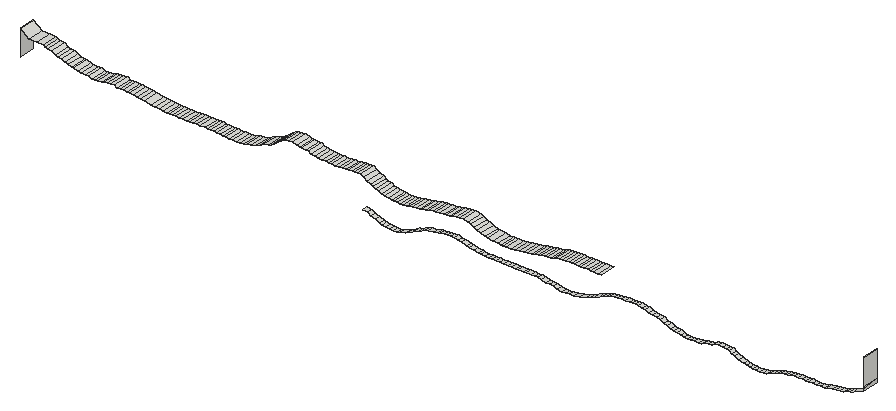
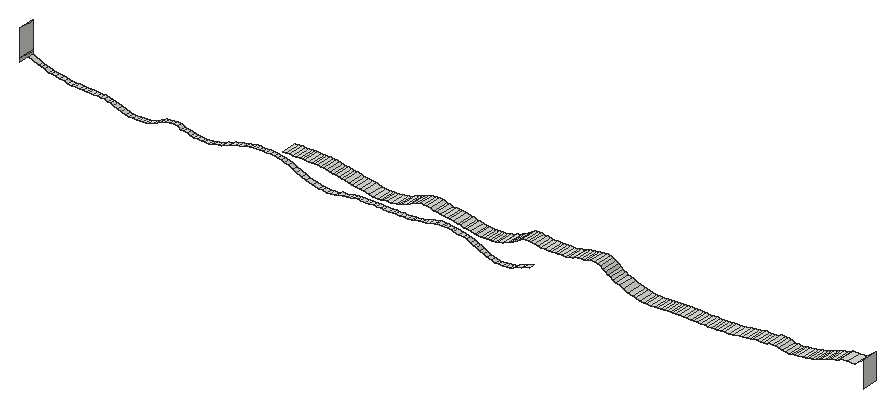
# SketchUp Ruby script. Lengths in inches.
U = 1.inch
M = Sketchup.active_model
def pt(a) = Geom::Point3d.new(a.map { |v| v * U })
def face(e, loops, mat)
  f = e.add_face(loops[0].map { |a| pt(a) })
  loops[1..].each { |l| e.add_face(l.map { |a| pt(a) }).erase! }
  f.material = f.back_material = mat if mat
  f
end
# faces: each face lists its corners as indices into pts; further lists are holes
def faces(e, pts, list, mat = nil) = list.each { |f| face(e, (f[0].is_a?(Array) ? f : [f]).map { |l| l.map { |i| pts[i] } }, mat) }
# xy, xz, yz: faces in a plane at the given z, y or x. An outline is a flat list of corners, or four numbers for a rectangle; further outlines are holes
def ring(l) = l.size == 4 ? [[l[0], l[1]], [l[2], l[1]], [l[2], l[3]], [l[0], l[3]]] : l.each_slice(2).to_a
def flat(e, list, mat, &to3) = list.each { |f| face(e, (f[0].is_a?(Array) ? f : [f]).map { |l| ring(l).map { |u, v| to3.(u, v) } }, mat) }
def xy(e, z, list, mat = nil) = flat(e, list, mat) { |x, y| [x, y, z] }
def xz(e, y, list, mat = nil) = flat(e, list, mat) { |x, z| [x, y, z] }
def yz(e, x, list, mat = nil) = flat(e, list, mat) { |y, z| [x, y, z] }
def lines(e, pts, list) = list.each { |a, b| e.add_line(pt(pts[a]), pt(pts[b])) }
# prism: a flat outline (further loops are holes) pulled along v
def prism(e, loops, v, mat = nil)
  f = face(e, loops, mat); d = Geom::Vector3d.new(v.map { |x| x * U })
  f.pushpull(f.normal.samedirection?(d) ? d.length : -d.length)
end
def box(e, o, s, mat = nil) = prism(e, [[o, [o[0] + s[0], o[1], o[2]], [o[0] + s[0], o[1] + s[1], o[2]], [o[0], o[1] + s[1], o[2]]]], [0, 0, s[2]], mat)
def at(x, y, z, deg = 0) = Geom::Transformation.translation(pt([x, y, z])) * Geom::Transformation.rotation(ORIGIN, Z_AXIS, deg.degrees)
def axes(o, x, y, z) = Geom::Transformation.new([*x, 0, *y, 0, *z, 0, *pt(o).to_a, 1])
def part(name) = M.definitions.add(name)
# library, detail: a bought-in or finely detailed component or shape, given as its bounding box
def library(name, o, s) = part(name).tap { |d| box(d.entities, o, s) }
def detail(e, o, s) = box(e.add_group.entities, o, s)
def put(e, d, t, mat = nil) = e.add_instance(d, t).tap { |i| i.material = mat if mat }
def group(e, t, mat = nil) = e.add_group.tap { |g| g.transformation = t; g.material = mat if mat }.entities
root = M.entities
xy(root,238.18,[[3012.28,2401.37,3012.96,2402.3]])
xy(root,238.62,[[2978.81,2401.37,2979.58,2402.3],[2979.58,2401.37,2980.21,2402.3],[2980.21,2401.37,2980.97,2402.3],[2980.97,2401.37,2981.59,2402.3],[2981.59,2401.37,2982.44,2402.3],
  [2982.44,2401.37,2983.08,2402.3],[2983.08,2401.37,2983.7,2402.3]])
xy(root,238.625,[[2977.39,2401.37,2978.25,2402.3]])
xy(root,238.89,[[3033.2,2401.37,3033.88,2402.3]])
xy(root,238.9,[[3034.64,2401.37,3035.26,2402.3],[3035.26,2401.37,3036.03,2402.3]])
xy(root,240.43,[[3001.48,2401.37,3002.05,2402.3]])
xy(root,241.68,[[2919.53,2401.37,2920.12,2404.3]])
xy(root,241.75,[[2921.88,2401.37,2922.75,2404.3],[2922.75,2401.37,2923.37,2404.3],[2923.37,2401.37,2923.88,2404.3]])
xy(root,243.05,[[2994.54,2401.37,2995.22,2404.3]])
xy(root,243.07,[[2992.6875,2401.37,2993.27,2404.3]])
xy(root,243.09,[[2989.375,2401.37,2989.9,2404.3],[2989.9,2401.37,2990.42,2404.3],[2990.42,2401.37,2991.08,2404.3],[2991.08,2401.37,2991.53,2404.3]])
yz(root,2889.09,[[2401.37,241.52,2404.3,246.2]])
yz(root,3043.1,[[2401.37,240.89,2401.37,241.29,2404.3,241.52,2404.3,240.89],[2401.37,241.29,2404.3,241.52,2401.37,241.52],[2401.37,241.52,2401.37,246.27,2402.0625,246.36,2404.3,246.43,2404.3,241.52],[2401.37,246.27,2401.37,246.43,2404.3,246.43,2402.0625,246.36]])
p = [[2955.89,2401.37,237.11],[2955.89,2402.3,237.11],[2956.65,2402.3,237.04],[2956.65,2401.37,237.04],[2957.34,2402.3,237.01],[2957.34,2401.37,237.01],
  [2957.95,2402.3,236.98],[2957.95,2401.37,236.98],[2958.63,2402.3,237.22],[2958.63,2401.37,237.22],[2955.2,2401.37,237.2],[2955.2,2402.3,237.2],
  [2954.67,2401.37,237.33],[2954.67,2402.3,237.33],[2959.48,2402.3,237.43],[2959.48,2401.37,237.43],[2954,2401.37,237.68],[2954,2402.3,237.68],
  [2960.1,2402.3,237.74],[2960.1,2401.37,237.74],[3022.93,2401.37,237.45],[3022.93,2402.3,237.45],[3023.5,2402.3,237.42],[3023.5,2401.37,237.42],
  [3024.23,2402.3,237.4],[3024.23,2401.37,237.4],[3024.91,2402.3,237.47],[3024.91,2401.37,237.47],[3021.74,2401.37,237.59],[3021.74,2402.3,237.59],
  [3022.34,2402.3,237.51],[3022.34,2401.37,237.51],[3025.51,2402.3,237.5625],[3025.51,2401.37,237.5625],[3021.2,2401.37,237.71],[3021.2,2402.3,237.71],
  [3026.2,2402.3,237.84],[3026.2,2401.37,237.84],[2953.0625,2401.37,237.96],[2953.0625,2402.3,237.96],[2960.8,2402.3,238.02],[2960.8,2401.37,238.02],
  [2987.94,2401.37,237.79],[2987.94,2402.3,237.79],[2988.65,2402.3,237.74],[2988.65,2401.37,237.74],[2989.52,2402.3,237.87],[2989.52,2401.37,237.87],
  [3020.37,2401.37,238],[3020.37,2402.3,238],[2987.17,2401.37,237.86],[2987.17,2402.3,237.86],[3026.88,2402.3,238.08],[3026.88,2401.37,238.08],
  [2986.54,2401.37,238.15],[2986.54,2402.3,238.15],[2990.17,2402.3,237.88],[2990.17,2401.37,237.88],[2991.29,2402.3,238.14],[2991.29,2401.37,238.14],
  [2952.5,2401.37,238.28],[2952.5,2402.3,238.28],[2961.24,2402.3,238.375],[2961.24,2401.37,238.375],[3019.66,2401.37,238.33],[3019.66,2402.3,238.33],
  [2985.77,2401.37,238.19],[2985.77,2402.3,238.19],[2992.51,2402.3,238.46],[2992.51,2401.37,238.46],[3010.26,2401.37,238.19],[3010.26,2402.3,238.19],
  [3011.08,2402.3,238.15],[3011.08,2401.37,238.15],[3011.61,2402.3,238.11],[3011.61,2401.37,238.11],[3012.28,2402.3,238.18],[3012.28,2401.37,238.18],
  [3027.57,2402.3,238.33],[3027.57,2401.37,238.33],[2985.15,2401.37,238.25],[2985.15,2402.3,238.25],[3009.6875,2401.37,238.26],[3009.6875,2402.3,238.26],
  [3012.96,2401.37,238.18],[3012.96,2402.3,238.18],[3013.64,2402.3,238.27],[3013.64,2401.37,238.27],[2951.72,2401.37,238.43],[2951.72,2402.3,238.43],
  [2984.39,2401.37,238.45],[2984.39,2402.3,238.45],[3009.12,2401.37,238.48],[3009.12,2402.3,238.48],[3014.16,2402.3,238.55],[3014.16,2401.37,238.55],
  [3019.11,2401.37,238.57],[3019.11,2402.3,238.57],[3028.1,2402.3,238.51],[3028.1,2401.37,238.51],[2961.8,2402.3,238.51],[2961.8,2401.37,238.51],
  [2962.4375,2402.3,238.76],[2962.4375,2401.37,238.76],[2983.7,2401.37,238.62],[2983.7,2402.3,238.62],[2993.26,2402.3,238.72],[2993.26,2401.37,238.72],
  [3008.46,2401.37,238.56],[3008.46,2402.3,238.56],[3014.82,2402.3,238.61],[3014.82,2401.37,238.61],[3028.67,2402.3,238.6],[3028.67,2401.37,238.6],
  [2974.63,2401.37,238.66],[2974.63,2402.3,238.66],[2975.3,2402.3,238.65],[2975.3,2401.37,238.65],[2976.08,2402.3,238.64],[2976.08,2401.37,238.64],
  [2976.7,2402.3,238.63],[2976.7,2401.37,238.63],[2977.39,2402.3,238.625],[2977.39,2401.37,238.625],[2978.25,2401.37,238.625],[2978.25,2402.3,238.625],
  [2978.81,2402.3,238.62],[2978.81,2401.37,238.62],[3007.89,2401.37,238.67],[3007.89,2402.3,238.67],[3015.41,2402.3,238.66],[3015.41,2401.37,238.66],
  [3018.61,2401.37,238.86],[3018.61,2402.3,238.86],[3029.33,2402.3,238.74],[3029.33,2401.37,238.74],[2972.79,2401.37,238.78],[2972.79,2402.3,238.78],
  [2973.27,2402.3,238.73],[2973.27,2401.37,238.73],[2973.94,2402.3,238.6875],[2973.94,2401.37,238.6875],[2994.14,2402.3,239.08],[2994.14,2401.37,239.08],
  [3007.37,2401.37,239.01],[3007.37,2402.3,239.01],[3015.98,2402.3,239.04],[3015.98,2401.37,239.04],[3029.91,2402.3,238.8],[3029.91,2401.37,238.8],
  [2963.08,2402.3,239.12],[2963.08,2401.37,239.12],[2971.91,2401.37,238.93],[2971.91,2402.3,238.93],[3030.48,2402.3,238.83],[3030.48,2401.37,238.83],
  [3031.22,2402.3,238.86],[3031.22,2401.37,238.86],[2971.14,2401.37,239.07],[2971.14,2402.3,239.07],[3018.09,2401.37,238.96],[3018.09,2402.3,238.96],
  [3031.98,2402.3,238.875],[3031.98,2401.37,238.875],[3032.52,2402.3,238.88],[3032.52,2401.37,238.88],[3033.2,2402.3,238.89],[3033.2,2401.37,238.89],
  [3033.88,2401.37,238.89],[3033.88,2402.3,238.89],[3034.64,2402.3,238.9],[3034.64,2401.37,238.9],[3036.03,2401.37,238.9],[3036.03,2402.3,238.9],
  [3036.66,2402.3,239.15],[3036.66,2401.37,239.15],[3006.6875,2401.37,239.18],[3006.6875,2402.3,239.18],[3016.72,2402.3,239.125],[3016.72,2401.37,239.125],
  [3017.4,2402.3,239.02],[3017.4,2401.37,239.02],[2963.66,2402.3,239.22],[2963.66,2401.37,239.22],[2970.59,2401.37,239.16],[2970.59,2402.3,239.16],
  [2994.93,2402.3,239.375],[2994.93,2401.37,239.375],[2964.66,2402.3,239.31],[2964.66,2401.37,239.31],[2969.74,2401.37,239.44],[2969.74,2402.3,239.44],
  [3006.0625,2401.37,239.5],[3006.0625,2402.3,239.5],[3037.43,2402.3,239.28],[3037.43,2401.37,239.28],[2965.47,2402.3,239.54],[2965.47,2401.37,239.54],
  [3038.23,2402.3,239.42],[3038.23,2401.37,239.42],[2969.07,2401.37,239.56],[2969.07,2402.3,239.56],[2995.67,2402.3,239.75],[2995.67,2401.37,239.75],
  [3038.95,2402.3,239.49],[3038.95,2401.37,239.49],[2965.96,2402.3,239.6],[2965.96,2401.37,239.6],[3005.3,2401.37,239.65],[3005.3,2402.3,239.65],
  [3039.5,2402.3,239.53],[3039.5,2401.37,239.53],[3040.1875,2402.3,239.81],[3040.1875,2401.37,239.81],[2966.58,2402.3,239.65],[2966.58,2401.37,239.65],
  [2967.17,2402.3,239.69],[2967.17,2401.37,239.69],[2968.46,2401.37,239.72],[2968.46,2402.3,239.72],[2967.73,2402.3,239.7],[2967.73,2401.37,239.7],
  [2996.32,2402.3,239.97],[2996.32,2401.37,239.97],[3004.6875,2401.37,239.8],[3004.6875,2402.3,239.8],[3003.93,2401.37,239.96],[3003.93,2402.3,239.96],
  [3040.71,2402.3,239.96],[3040.71,2401.37,239.96],[2996.94,2402.3,240.17],[2996.94,2401.37,240.17],[3003.28,2401.37,240.23],[3003.28,2402.3,240.23],
  [3041.27,2402.3,240.1],[3041.27,2401.37,240.1],[3043.1,2402.3,240.89],[3043.1,2401.37,240.89],[2997.62,2402.3,240.27],[2997.62,2401.37,240.27],
  [3002.7,2401.37,240.27],[3002.7,2402.3,240.27],[2998.3,2402.3,240.33],[2998.3,2401.37,240.33],[2998.99,2402.3,240.37],[2998.99,2401.37,240.37],
  [3002.05,2401.37,240.43],[3002.05,2402.3,240.43],[2999.68,2402.3,240.4],[2999.68,2401.37,240.4],[3000.375,2402.3,240.41],[3000.375,2401.37,240.41],
  [3000.9,2402.3,240.42],[3000.9,2401.37,240.42],[3001.48,2402.3,240.43],[3001.48,2401.37,240.43],[2925.51,2404.3,241.57],[2926.05,2404.3,241.53],
  [2926.05,2401.37,241.53],[2925.51,2401.37,241.57],[2926.67,2404.3,241.51],[2926.67,2401.37,241.51],[2927.22,2404.3,241.49],[2927.22,2401.37,241.49],
  [2927.92,2404.3,241.48],[2927.92,2401.37,241.48],[2928.58,2404.3,241.47],[2928.58,2401.37,241.47],[2929.15,2404.3,241.46],[2929.15,2401.37,241.46],
  [2929.86,2404.3,241.6],[2929.86,2401.37,241.6],[2976.23,2404.3,241.56],[2976.83,2404.3,241.51],[2976.83,2401.37,241.51],[2976.23,2401.37,241.56],
  [2977.28,2404.3,241.48],[2977.28,2401.37,241.48],[2977.8,2404.3,241.46],[2977.8,2401.37,241.46],[2978.67,2404.3,241.51],[2978.67,2401.37,241.51],
  [2979.39,2404.3,241.59],[2979.39,2401.37,241.59],[2924.9,2404.3,241.66],[2924.9,2401.37,241.66],[2930.59,2404.3,241.85],[2930.59,2401.37,241.85],
  [2974.41,2404.3,241.78],[2975.46,2404.3,241.63],[2975.46,2401.37,241.63],[2974.41,2401.37,241.78],[2980.33,2404.3,241.82],[2980.33,2401.37,241.82],
  [2915.87,2404.3,241.75],[2916.32,2404.3,241.74],[2916.32,2401.37,241.74],[2915.87,2401.37,241.75],[2916.87,2404.3,241.72],[2916.87,2401.37,241.72],
  [2917.5,2404.3,241.71],[2917.5,2401.37,241.71],[2918.13,2404.3,241.7],[2918.13,2401.37,241.7],[2918.86,2404.3,241.69],[2918.86,2401.37,241.69],
  [2919.53,2404.3,241.68],[2919.53,2401.37,241.68],[2920.12,2404.3,241.68],[2920.61,2404.3,241.67],[2920.61,2401.37,241.67],[2920.12,2401.37,241.68],
  [2921.3125,2404.3,241.74],[2921.3125,2401.37,241.74],[2921.88,2404.3,241.75],[2921.88,2401.37,241.75],[2923.88,2404.3,241.75],[2924.37,2404.3,241.67],
  [2924.37,2401.37,241.67],[2923.88,2401.37,241.75],[2913.68,2404.3,241.89],[2914.5,2404.3,241.83],[2914.5,2401.37,241.83],[2913.68,2401.37,241.89],
  [2915.1,2404.3,241.78],[2915.1,2401.37,241.78],[2931.26,2404.3,241.91],[2931.26,2401.37,241.91],[2956.89,2404.3,241.89],[2957.35,2404.3,241.85],
  [2957.35,2401.37,241.85],[2956.89,2401.37,241.89],[2957.87,2404.3,241.8125],[2957.87,2401.37,241.8125],[2958.38,2404.3,241.79],[2958.38,2401.37,241.79],
  [2958.96,2404.3,241.78],[2958.96,2401.37,241.78],[2959.63,2404.3,241.91],[2959.63,2401.37,241.91],[2973.92,2404.3,241.89],[2973.92,2401.37,241.89],
  [2981.11,2404.3,241.87],[2981.11,2401.37,241.87],[2912.91,2404.3,241.96],[2912.91,2401.37,241.96],[2932.16,2404.3,242.1],[2932.16,2401.37,242.1],
  [2956.33,2404.3,241.96],[2956.33,2401.37,241.96],[2960.1,2404.3,241.93],[2960.1,2401.37,241.93],[2960.77,2404.3,242.09],[2960.77,2401.37,242.09],
  [2973.28,2404.3,242.14],[2973.28,2401.37,242.14],[2981.875,2404.3,241.98],[2981.875,2401.37,241.98],[2911.74,2404.3,242.24],[2911.74,2401.37,242.24],
  [2955.65,2404.3,242.11],[2955.65,2401.37,242.11],[2982.49,2404.3,242.02],[2982.49,2401.37,242.02],[2983.14,2404.3,242.19],[2983.14,2401.37,242.19],
  [2932.93,2404.3,242.46],[2932.93,2401.37,242.46],[2955.05,2404.3,242.21],[2955.05,2401.37,242.21],[2961.54,2404.3,242.2],[2961.54,2401.37,242.2],
  [2972.52,2404.3,242.39],[2972.52,2401.37,242.39],[2911.07,2404.3,242.34],[2911.07,2401.37,242.34],[2954.54,2404.3,242.51],[2954.54,2401.37,242.51],
  [2962.04,2404.3,242.24],[2962.04,2401.37,242.24],[2962.65,2404.3,242.42],[2962.65,2401.37,242.42],[2983.84,2404.3,242.38],[2983.84,2401.37,242.38],
  [2910.41,2404.3,242.38],[2910.41,2401.37,242.38],[2909.75,2404.3,242.48],[2909.75,2401.37,242.48],[2963.2,2404.3,242.47],[2963.2,2401.37,242.47],
  [2971.9,2404.3,242.65],[2971.9,2401.37,242.65],[2984.33,2404.3,242.4375],[2984.33,2401.37,242.4375],[2984.85,2404.3,242.48],[2984.85,2401.37,242.48],
  [2901.57,2404.3,242.68],[2902.24,2404.3,242.51],[2902.24,2401.37,242.51],[2901.57,2401.37,242.68],[2902.76,2404.3,242.46],[2902.76,2401.37,242.46],
  [2903.3,2404.3,242.58],[2903.3,2401.37,242.58],[2909.11,2404.3,242.57],[2909.11,2401.37,242.57],[2933.63,2404.3,242.78],[2933.63,2401.37,242.78],
  [2953.95,2404.3,242.68],[2953.95,2401.37,242.68],[2963.95,2404.3,242.71],[2963.95,2401.37,242.71],[2985.51,2404.3,242.58],[2985.51,2401.37,242.58],
  [2903.93,2404.3,242.57],[2903.93,2401.37,242.57],[2904.56,2404.3,242.81],[2904.56,2401.37,242.81],[2906.33,2404.3,242.92],[2906.76,2404.3,242.625],
  [2906.76,2401.37,242.625],[2906.33,2401.37,242.92],[2907.37,2404.3,242.65],[2907.37,2401.37,242.65],[2907.92,2404.3,242.62],[2907.92,2401.37,242.62],
  [2908.55,2404.3,242.58],[2908.55,2401.37,242.58],[2971.35,2404.3,242.9375],[2971.35,2401.37,242.9375],[2986.04,2404.3,242.61],[2986.04,2401.37,242.61],
  [2986.625,2404.3,242.77],[2986.625,2401.37,242.77],[2900.22,2404.3,242.78],[2901.03,2404.3,242.73],[2901.03,2401.37,242.73],[2900.22,2401.37,242.78],
  [2953.45,2404.3,242.875],[2953.45,2401.37,242.875],[2964.59,2404.3,242.78],[2964.59,2401.37,242.78],[2898.92,2404.3,243.06],[2899.64,2404.3,242.85],
  [2899.64,2401.37,242.85],[2898.92,2401.37,243.06],[2905.13,2404.3,242.86],[2905.13,2401.37,242.86],[2934.4,2404.3,242.97],[2934.4,2401.37,242.97],
  [2965.07,2404.3,242.82],[2965.07,2401.37,242.82],[2965.76,2404.3,242.85],[2965.76,2401.37,242.85],[2987.08,2404.3,242.95],[2987.08,2401.37,242.95],
  [2905.69,2404.3,242.89],[2905.69,2401.37,242.89],[2953.06,2404.3,243.09],[2953.06,2401.37,243.09],[2966.46,2404.3,242.87],[2966.46,2401.37,242.87],
  [2967.01,2404.3,243.02],[2967.01,2401.37,243.02],[2970.78,2404.3,243.14],[2970.78,2401.37,243.14],[2934.93,2404.3,243.23],[2934.93,2401.37,243.23],
  [2967.63,2404.3,243.05],[2967.63,2401.37,243.05],[2987.64,2404.3,243.01],[2987.64,2401.37,243.01],[2988.15,2404.3,243.05],[2988.15,2401.37,243.05],
  [2988.72,2404.3,243.08],[2988.72,2401.37,243.08],[2897.85,2404.3,243.3],[2898.4375,2404.3,243.14],[2898.4375,2401.37,243.14],[2897.85,2401.37,243.3],
  [2952.45,2404.3,243.43],[2952.45,2401.37,243.43],[2968.18,2404.3,243.29],[2968.18,2401.37,243.29],[2970.01,2404.3,243.42],[2970.01,2401.37,243.42],
  [2989.375,2404.3,243.09],[2989.375,2401.37,243.09],[2991.53,2404.3,243.09],[2992.1,2404.3,243.08],[2992.1,2401.37,243.08],[2991.53,2401.37,243.09],
  [2992.6875,2404.3,243.07],[2992.6875,2401.37,243.07],[2993.27,2404.3,243.07],[2993.93,2404.3,243.0625],[2993.93,2401.37,243.0625],[2993.27,2401.37,243.07],
  [2994.54,2404.3,243.05],[2994.54,2401.37,243.05],[2935.33,2404.3,243.48],[2935.33,2401.37,243.48],[2897.21,2404.3,243.48],[2897.21,2401.37,243.48],
  [2968.86,2404.3,243.35],[2968.86,2401.37,243.35],[2951.91,2404.3,243.8],[2951.91,2401.37,243.8],[2969.41,2404.3,243.39],[2969.41,2401.37,243.39],
  [2896.69,2404.3,243.79],[2896.69,2401.37,243.79],[2935.85,2404.3,243.72],[2935.85,2401.37,243.72],[2936.1875,2404.3,244.12],[2936.1875,2401.37,244.12],
  [2896.03,2404.3,243.95],[2896.03,2401.37,243.95],[2951.31,2404.3,244.18],[2951.31,2401.37,244.18],[2895.51,2404.3,244.11],[2895.51,2401.37,244.11],
  [2944.13,2404.3,243.99],[2944.85,2404.3,243.95],[2944.85,2401.37,243.95],[2944.13,2401.37,243.99],[2945.35,2404.3,243.93],[2945.35,2401.37,243.93],
  [2946.04,2404.3,243.91],[2946.04,2401.37,243.91],[2946.61,2404.3,243.89],[2946.61,2401.37,243.89],[2947.31,2404.3,243.88],[2947.31,2401.37,243.88],
  [2947.96,2404.3,243.94],[2947.96,2401.37,243.94],[2948.6,2404.3,243.95],[2948.6,2401.37,243.95],[2949.16,2404.3,244.1],[2949.16,2401.37,244.1],
  [2942.95,2404.3,244.11],[2943.51,2404.3,244.04],[2943.51,2401.37,244.04],[2942.95,2401.37,244.11],[2894.84,2404.3,244.41],[2894.84,2401.37,244.41],
  [2936.66,2404.3,244.39],[2936.66,2401.37,244.39],[2942.2,2404.3,244.25],[2942.2,2401.37,244.25],[2949.79,2404.3,244.13],[2949.79,2401.37,244.13],
  [2950.27,2404.3,244.15],[2950.27,2401.37,244.15],[2950.79,2404.3,244.17],[2950.79,2401.37,244.17],[2941.74,2404.3,244.51],[2941.74,2401.37,244.51],
  [2894.08,2404.3,244.54],[2894.08,2401.37,244.54],[2937.14,2404.3,244.73],[2937.14,2401.37,244.73],[2893.52,2404.3,244.61],[2893.52,2401.37,244.61],
  [2940.59,2404.3,244.67],[2941.2,2404.3,244.55],[2941.2,2401.37,244.55],[2940.59,2401.37,244.67],[2893.3,2404.3,244.92],[2893.3,2401.37,244.92],
  [2937.625,2404.3,244.87],[2937.625,2401.37,244.87],[2939.54,2404.3,244.81],[2940.11,2404.3,244.7],[2940.11,2401.37,244.7],[2939.54,2401.37,244.81],
  [2938.89,2404.3,245.01],[2938.89,2401.37,245.01],[2890.66,2404.3,244.96],[2892.05,2404.3,244.9375],[2892.05,2401.37,244.9375],[2890.66,2401.37,244.96],
  [2938.21,2404.3,244.95],[2938.21,2401.37,244.95],[2889.09,2404.3,246.2],[2889.09,2401.37,246.2]]
faces(root,p,[[0,1,2,3],[3,2,4,5],[5,4,6,7],[7,6,8,9],[10,11,1,0],[12,13,11,10],[9,8,14,15],[16,17,13,12],
  [15,14,18,19],[20,21,22,23],[23,22,24,25],[25,24,26,27],[28,29,30,31],[31,30,21,20],[27,26,32,33],[34,35,29,28],
  [33,32,36,37],[38,39,17,16],[19,18,40,41],[42,43,44,45],[45,44,46,47],[48,49,35,34],[50,51,43,42],[37,36,52,53],
  [54,55,51,50],[47,46,56,57],[57,56,58,59],[60,61,39,38],[41,40,62,63],[64,65,49,48],[66,67,55,54],[59,58,68,69],
  [70,71,72,73],[73,72,74,75],[75,74,76,77],[53,52,78,79],[80,81,67,66],[82,83,71,70],[84,85,86,87],[88,89,61,60],
  [90,91,81,80],[92,93,83,82],[87,86,94,95],[96,97,65,64],[79,78,98,99],[63,62,100,101],[101,100,102,103],[104,105,91,90],
  [69,68,106,107],[108,109,93,92],[95,94,110,111],[99,98,112,113],[114,115,116,117],[117,116,118,119],[119,118,120,121],[121,120,122,123],
  [124,125,126,127],[128,129,109,108],[111,110,130,131],[132,133,97,96],[113,112,134,135],[136,137,138,139],[139,138,140,141],[141,140,115,114],
  [107,106,142,143],[144,145,129,128],[131,130,146,147],[135,134,148,149],[103,102,150,151],[152,153,137,136],[149,148,154,155],[155,154,156,157],
  [158,159,153,152],[160,161,133,132],[157,156,162,163],[163,162,164,165],[165,164,166,167],[168,169,170,171],[172,173,174,175],[176,177,145,144],
  [147,146,178,179],[179,178,180,181],[181,180,161,160],[151,150,182,183],[184,185,159,158],[143,142,186,187],[183,182,188,189],[190,191,185,184],
  [192,193,177,176],[175,174,194,195],[189,188,196,197],[195,194,198,199],[200,201,191,190],[187,186,202,203],[199,198,204,205],[197,196,206,207],
  [208,209,193,192],[205,204,210,211],[211,210,212,213],[207,206,214,215],[215,214,216,217],[218,219,201,200],[217,216,220,221],[221,220,219,218],
  [203,202,222,223],[224,225,209,208],[226,227,225,224],[213,212,228,229],[223,222,230,231],[232,233,227,226],[229,228,234,235],[235,234,236,237],
  [231,230,238,239],[240,241,233,232],[239,238,242,243],[243,242,244,245],[246,247,241,240],[245,244,248,249],[249,248,250,251],[251,250,252,253],
  [253,252,254,255],[256,257,258,259],[257,260,261,258],[260,262,263,261],[262,264,265,263],[264,266,267,265],[266,268,269,267],[268,270,271,269],
  [272,273,274,275],[273,276,277,274],[276,278,279,277],[278,280,281,279],[280,282,283,281],[284,256,259,285],[270,286,287,271],[288,289,290,291],
  [289,272,275,290],[282,292,293,283],[294,295,296,297],[295,298,299,296],[298,300,301,299],[300,302,303,301],[302,304,305,303],[304,306,307,305],
  [308,309,310,311],[309,312,313,310],[312,314,315,313],[316,317,318,319],[317,284,285,318],[320,321,322,323],[321,324,325,322],[324,294,297,325],
  [286,326,327,287],[328,329,330,331],[329,332,333,330],[332,334,335,333],[334,336,337,335],[336,338,339,337],[340,288,291,341],[292,342,343,293],
  [344,320,323,345],[326,346,347,327],[348,328,331,349],[338,350,351,339],[350,352,353,351],[354,340,341,355],[342,356,357,343],[358,344,345,359],
  [360,348,349,361],[356,362,363,357],[362,364,365,363],[346,366,367,347],[368,360,361,369],[352,370,371,353],[372,354,355,373],[374,358,359,375],
  [376,368,369,377],[370,378,379,371],[378,380,381,379],[364,382,383,365],[384,374,375,385],[386,384,385,387],[380,388,389,381],[390,372,373,391],
  [382,392,393,383],[392,394,395,393],[396,397,398,399],[397,400,401,398],[400,402,403,401],[404,386,387,405],[366,406,407,367],[408,376,377,409],
  [388,410,411,389],[394,412,413,395],[402,414,415,403],[414,416,417,415],[418,419,420,421],[419,422,423,420],[422,424,425,423],[424,426,427,425],
  [426,404,405,427],[428,390,391,429],[412,430,431,413],[430,432,433,431],[434,435,436,437],[435,396,399,436],[438,408,409,439],[410,440,441,411],
  [442,443,444,445],[443,434,437,444],[416,446,447,417],[406,448,449,407],[440,450,451,441],[450,452,453,451],[432,454,455,433],[446,456,457,447],
  [456,418,421,457],[458,438,439,459],[452,460,461,453],[460,462,463,461],[464,428,429,465],[448,466,467,449],[462,468,469,463],[454,470,471,455],
  [470,472,473,471],[472,474,475,473],[476,477,478,479],[477,442,445,478],[480,458,459,481],[468,482,483,469],[484,464,465,485],[474,486,487,475],
  [488,489,490,491],[489,492,493,490],[494,495,496,497],[495,498,499,496],[466,500,501,467],[502,476,479,503],[482,504,505,483],[506,480,481,507],
  [504,508,509,505],[508,484,485,509],[510,502,503,511],[500,512,513,501],[512,514,515,513],[516,510,511,517],[518,506,507,519],[520,516,517,521],
  [522,523,524,525],[523,526,527,524],[526,528,529,527],[528,530,531,529],[530,532,533,531],[532,534,535,533],[534,536,537,535],[536,538,539,537],
  [540,541,542,543],[541,522,525,542],[544,520,521,545],[514,546,547,515],[548,540,543,549],[538,550,551,539],[550,552,553,551],[552,554,555,553],
  [554,518,519,555],[556,548,549,557],[558,544,545,559],[546,560,561,547],[562,558,559,563],[564,565,566,567],[565,556,557,566],[568,562,563,569],
  [560,570,571,561],[572,573,574,575],[573,564,567,574],[576,572,575,577],[578,579,580,581],[579,568,569,580],[570,582,583,571],[582,576,577,583],
  [584,578,581,585]])
